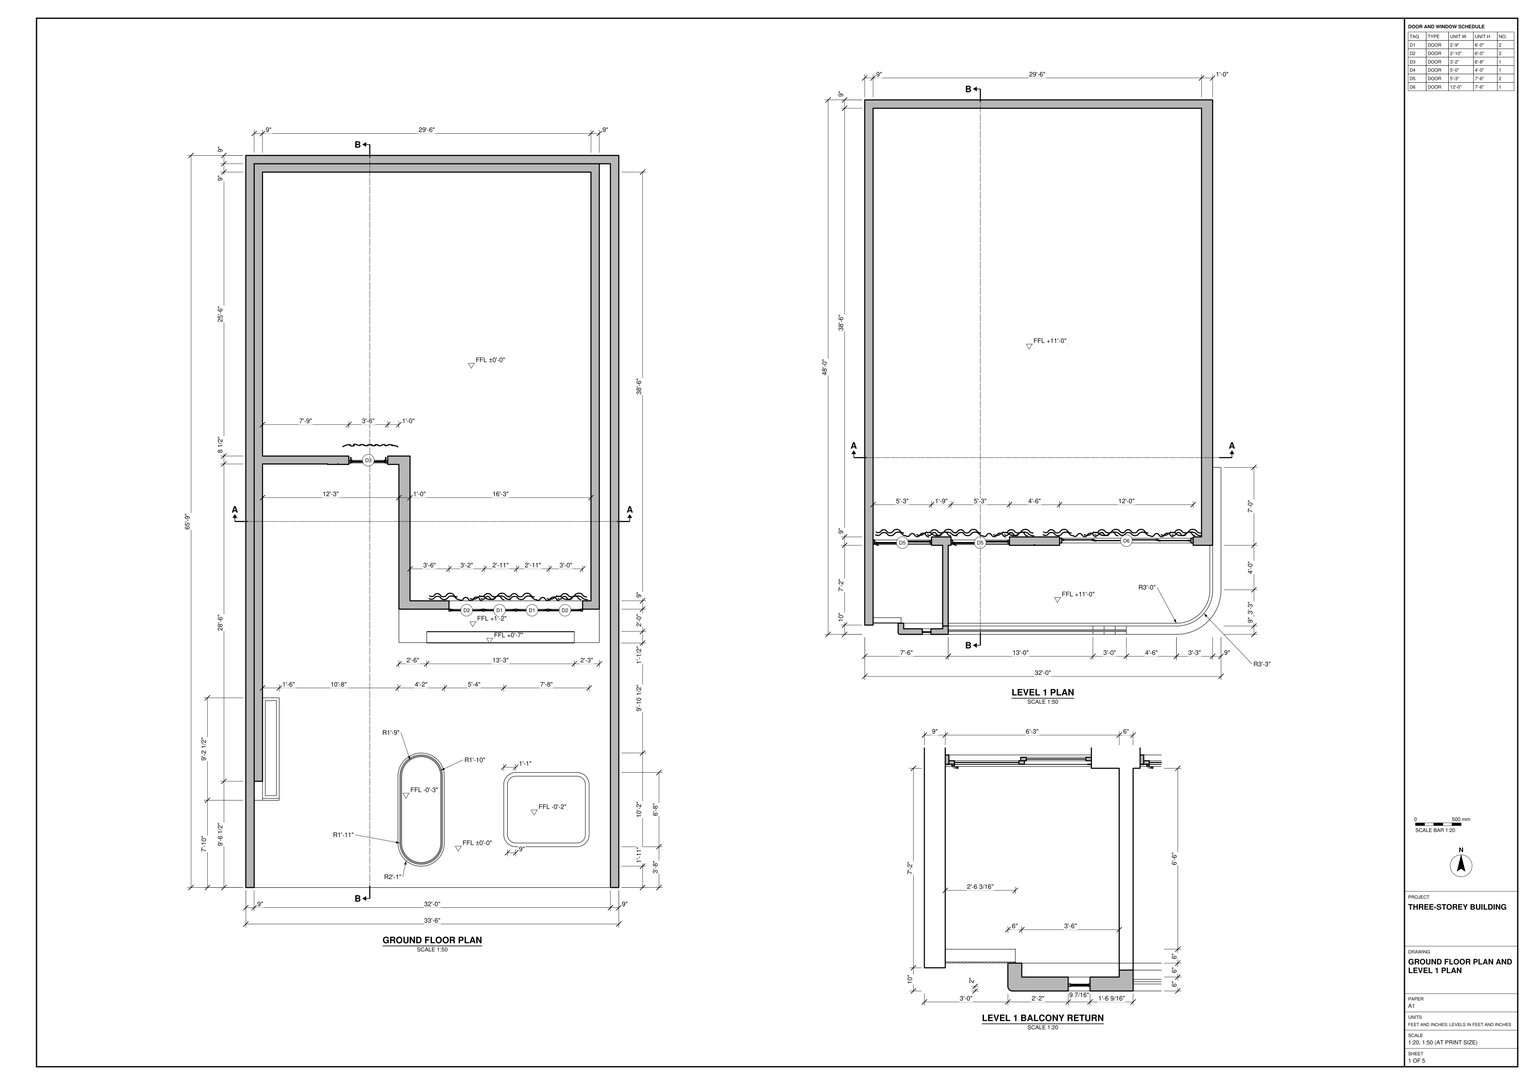
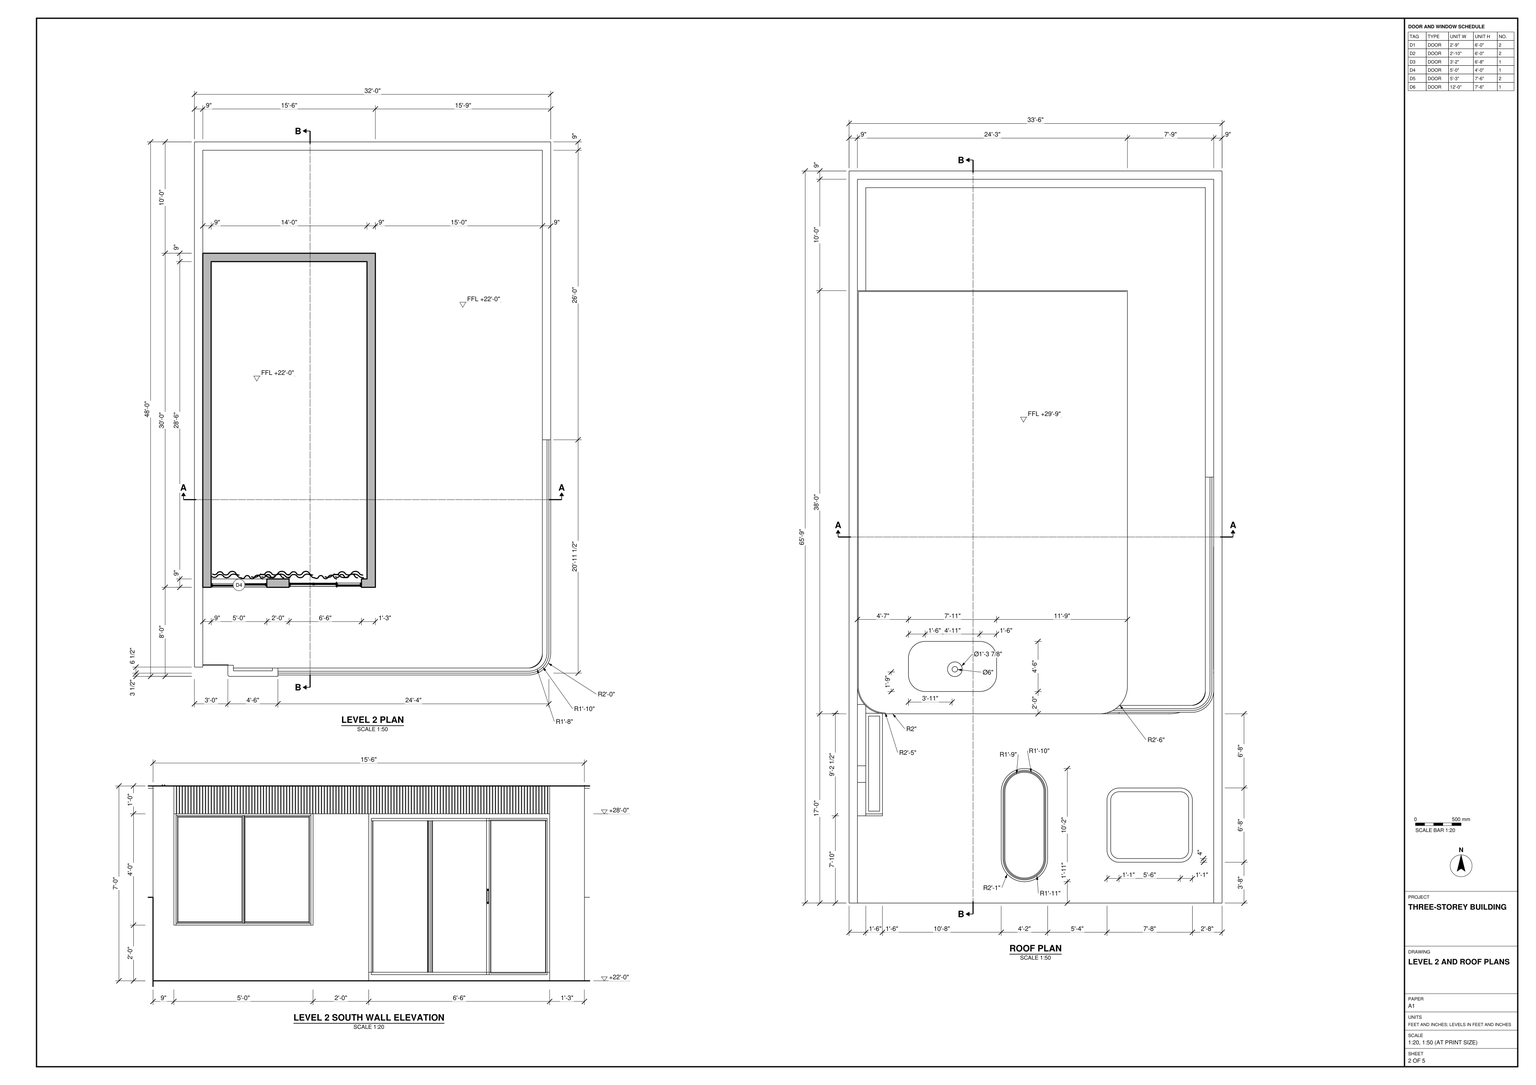
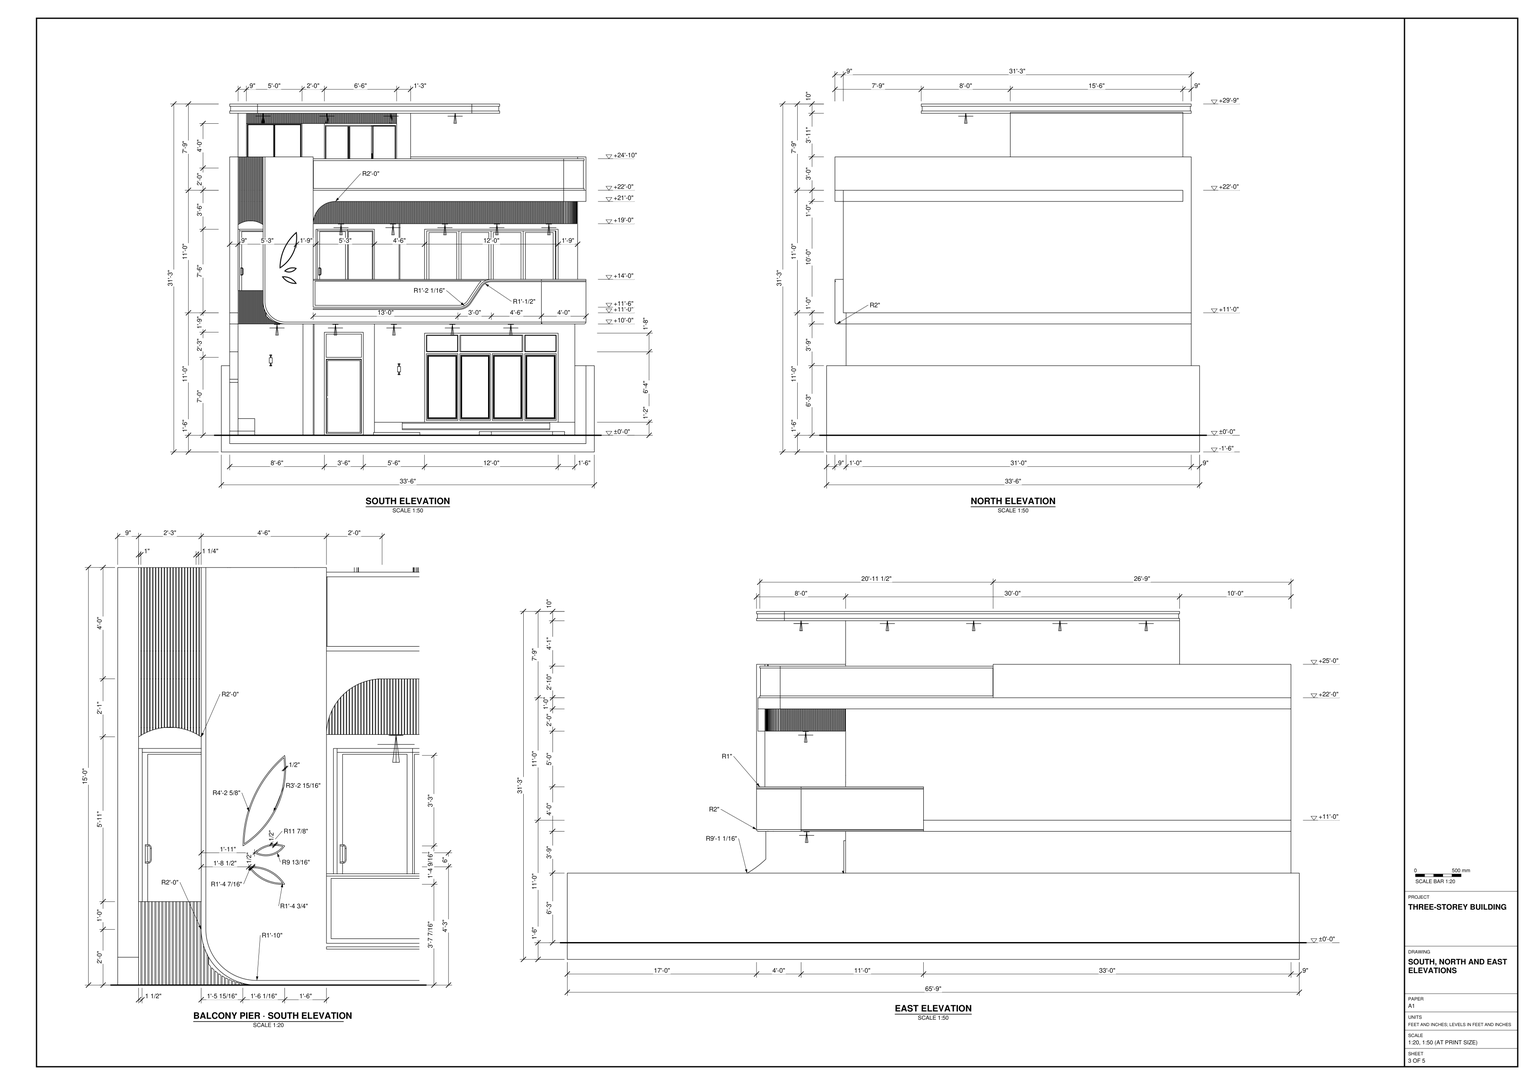
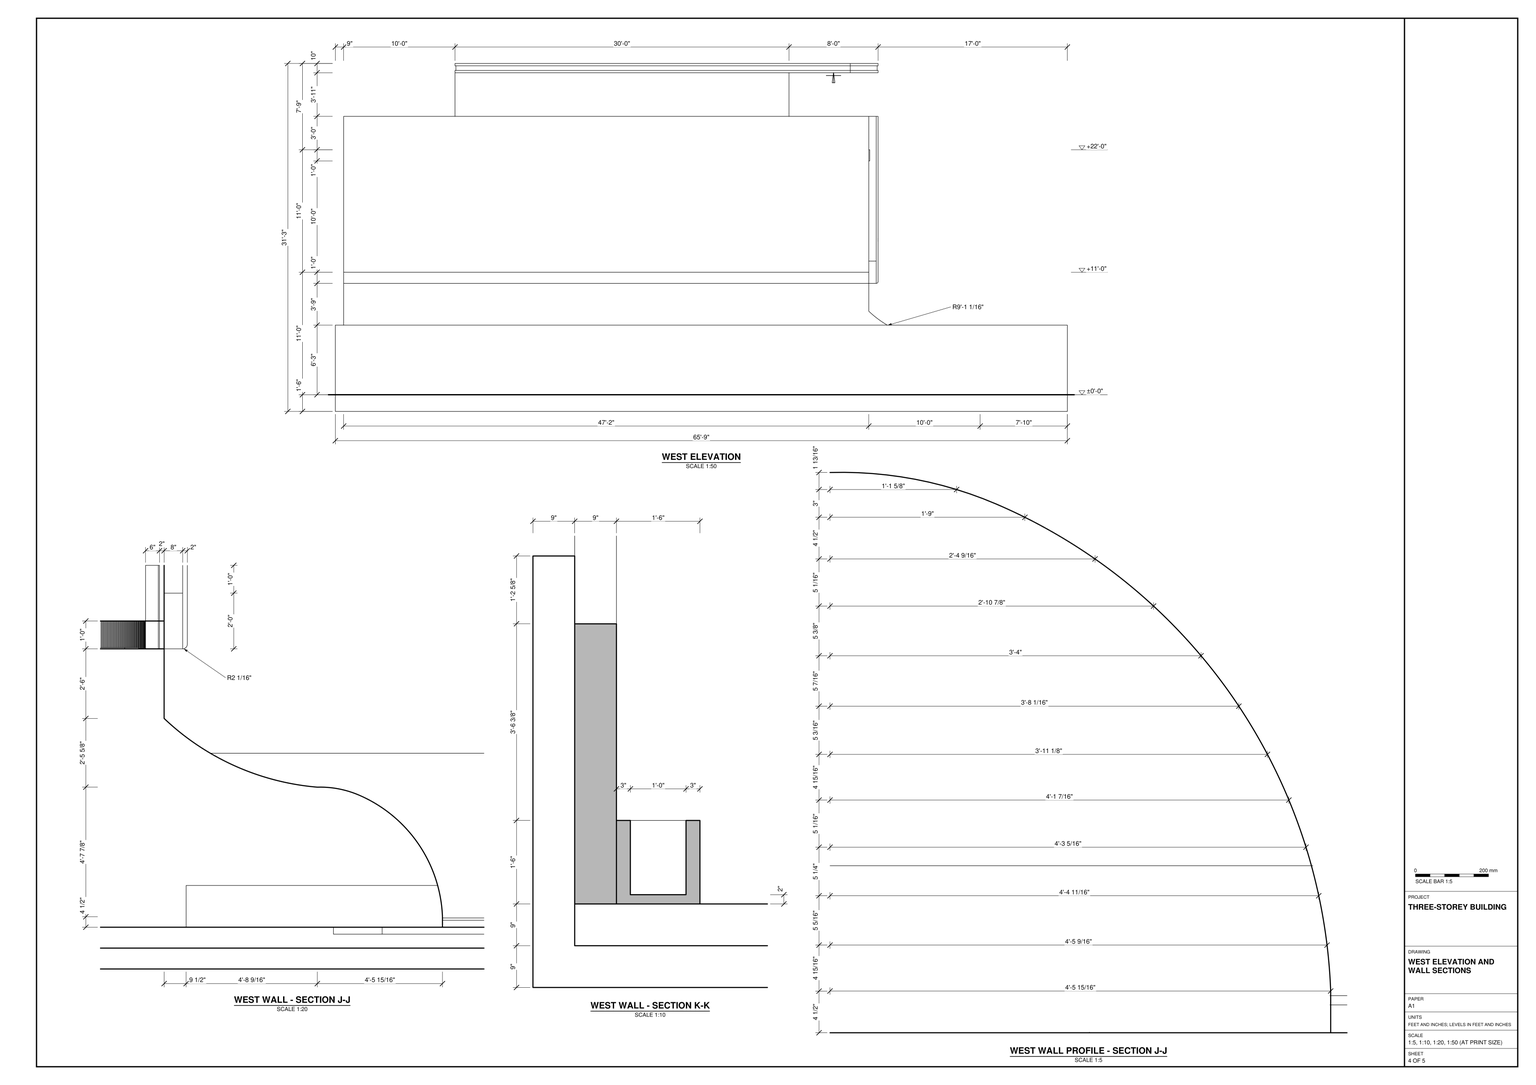
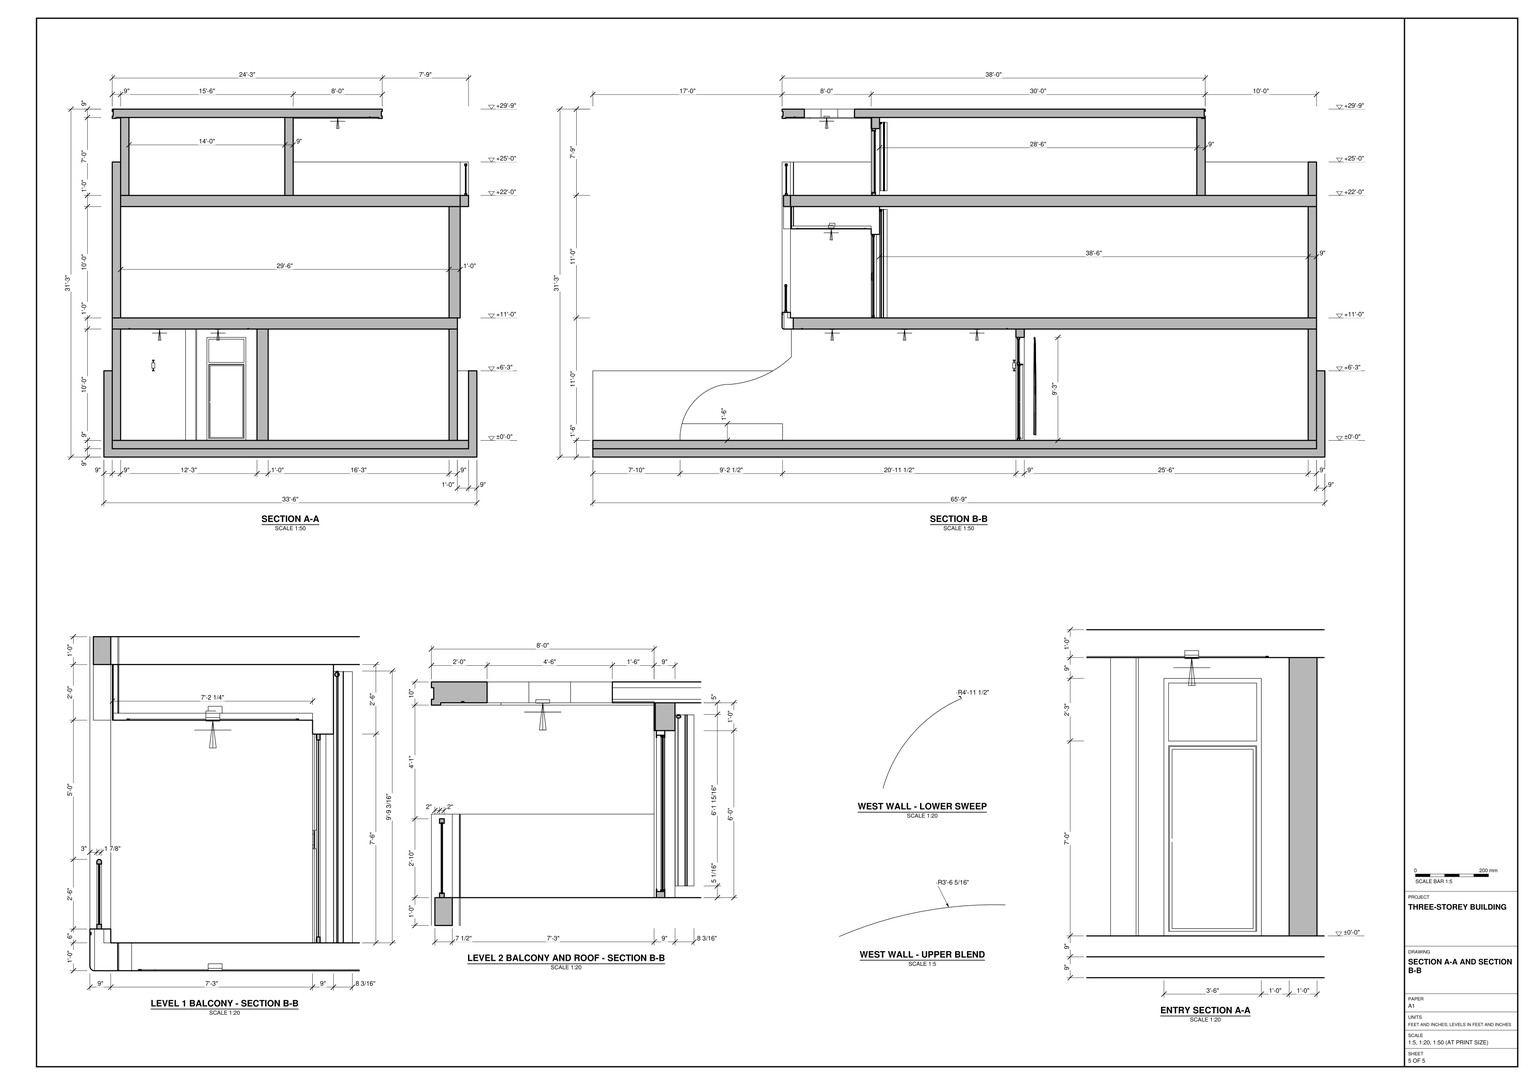
Build the three-storey building in SketchUp from task_files/diagram_01.pdf. Work in feet and inches. The overall dimensions, including the base and forecourt, are 33'-6" wide by 65'-9" deep by 31'-3" high. Set the finished floor levels to ±0'-0", +11'-0" and +22'-0". Include the base below the ground floor so the overall height matches the elevations.

Use the plans to lay out the walls at their drawn thicknesses, including the 9" wall runs and the 1'-0" return beside the recessed entrance. Model the forecourt, its side walls and its rounded inset features. Follow the door schedule and south elevation for the entrance, shallow steps, framed glazing and panels above the ground-floor openings.

At the middle storey, carry the balcony around the rounded front corner and shape its parapet and tall pier from the elevation details. Set the narrower top-storey enclosure back on the terrace and cover it with the projecting flat roof. Use the plans and elevations together to locate slab edges, parapets and openings.

Keep walls, slabs, roof and each furniture or joinery piece shown as separate groups or components, and use components for repeated parts. Decor and loose items may be any suitable library components. Save one SketchUp model as output_files/three_storey_building_curved_balcony_and_roof_terrace.skp.

# SketchUp Ruby script. Lengths in inches.
U = 1.inch
M = Sketchup.active_model
def pt(a) = Geom::Point3d.new(a.map { |v| v * U })
def face(e, loops, mat)
  f = e.add_face(loops[0].map { |a| pt(a) })
  loops[1..].each { |l| e.add_face(l.map { |a| pt(a) }).erase! }
  f.material = f.back_material = mat if mat
  f
end
# faces: each face lists its corners as indices into pts; further lists are holes
def faces(e, pts, list, mat = nil) = list.each { |f| face(e, (f[0].is_a?(Array) ? f : [f]).map { |l| l.map { |i| pts[i] } }, mat) }
# xy, xz, yz: faces in a plane at the given z, y or x. An outline is a flat list of corners, or four numbers for a rectangle; further outlines are holes
def ring(l) = l.size == 4 ? [[l[0], l[1]], [l[2], l[1]], [l[2], l[3]], [l[0], l[3]]] : l.each_slice(2).to_a
def flat(e, list, mat, &to3) = list.each { |f| face(e, (f[0].is_a?(Array) ? f : [f]).map { |l| ring(l).map { |u, v| to3.(u, v) } }, mat) }
def xy(e, z, list, mat = nil) = flat(e, list, mat) { |x, y| [x, y, z] }
def xz(e, y, list, mat = nil) = flat(e, list, mat) { |x, z| [x, y, z] }
def yz(e, x, list, mat = nil) = flat(e, list, mat) { |y, z| [x, y, z] }
def lines(e, pts, list) = list.each { |a, b| e.add_line(pt(pts[a]), pt(pts[b])) }
# prism: a flat outline (further loops are holes) pulled along v
def prism(e, loops, v, mat = nil)
  f = face(e, loops, mat); d = Geom::Vector3d.new(v.map { |x| x * U })
  f.pushpull(f.normal.samedirection?(d) ? d.length : -d.length)
end
def box(e, o, s, mat = nil) = prism(e, [[o, [o[0] + s[0], o[1], o[2]], [o[0] + s[0], o[1] + s[1], o[2]], [o[0], o[1] + s[1], o[2]]]], [0, 0, s[2]], mat)
def at(x, y, z, deg = 0) = Geom::Transformation.translation(pt([x, y, z])) * Geom::Transformation.rotation(ORIGIN, Z_AXIS, deg.degrees)
def axes(o, x, y, z) = Geom::Transformation.new([*x, 0, *y, 0, *z, 0, *pt(o).to_a, 1])
def part(name) = M.definitions.add(name)
# library, detail: a bought-in or finely detailed component or shape, given as its bounding box
def library(name, o, s) = part(name).tap { |d| box(d.entities, o, s) }
def detail(e, o, s) = box(e.add_group.entities, o, s)
def put(e, d, t, mat = nil) = e.add_instance(d, t).tap { |i| i.material = mat if mat }
def group(e, t, mat = nil) = e.add_group.tap { |g| g.transformation = t; g.material = mat if mat }.entities
root = M.entities
M.materials.add("0027 AP L140 CRUSHED ICE").color = [241, 233, 217]
M.materials.add("Black_matte").color = [7, 7, 7]
M.materials.add("Carpet_Frieze_Low").color = [170, 156, 146]
M.materials.add("Carpet_Loop_Low").color = [201, 172, 127]
M.materials.add("Glass_Tinted_Gray").color = [0, 0, 0]
M.materials.add("Glass_headlight").color = [127, 127, 127]
M.materials.add("[0135_DarkGray]").color = [81, 81, 81]
M.materials.add("[Mirror 02]").color = [229, 229, 229]
M.materials.add("[Terrazzo Light Blue]").color = [196, 214, 227]
M.materials.add("[Wood Cherry Original]").color = [103, 58, 28]
c1 = library("CURTAIN",[20.4,9.88,0],[29.77,2.88,102.36])
c2 = library("Sliding glass door",[0,0,0],[5.83,106.3,82.68])
c3 = part("PENTEK_RP Fineline 50S_Sliding_DoorCase_E1")
box(c3.entities,[0,0,0],[1.51,3.66,99.27],"[0135_DarkGray]")
c4 = part("PENTEK_RP Fineline 50S_SlidingDooe_Case_E2")
box(c4.entities,[0,0,0],[96.25,3.66,1.51],"[0135_DarkGray]")
c5 = part("pentek_RP Fineline 50S_SlidingDoor_Case")
put(c5.entities,c3,at(97.76,0,0))
put(c5.entities,c4,at(1.51,0,0))
put(c5.entities,c3,at(0,0,0))
put(c5.entities,c4,at(1.51,0,97.76))
c6 = part("PENTEK_RP Fineline 50S_SlidingDoor_GlazingBead_2")
box(c6.entities,[0,0,0],[0.56,0.59,94.39],"[0135_DarkGray]")
c7 = part("PENTEK_RP Fineline 50S_SlidingDoor_Glass")
box(c7.entities,[0,0,0],[46.58,0.16,94.39],"Glass_Tinted_Gray")
c8 = part("PENTEK_RP Fineline 50S_SlidingDoor_GlazingBead")
box(c8.entities,[0,0,0],[45.47,0.59,0.56],"[0135_DarkGray]")
c9 = part("PENTEK_RP Fineline 50S_SlidingDoor_Leaf_E1")
xy(c9.entities,0,[[0,0,0.93,1.97],[0.93,1.57,1.49,1.97]],"[0135_DarkGray]")
xy(c9.entities,96.25,[[0,0,0.93,0,0.93,1.57,1.49,1.57,1.49,1.97,0,1.97]],"[0135_DarkGray]")
xz(c9.entities,0,[[0,0,0.93,96.25]],"[0135_DarkGray]")
xz(c9.entities,1.57,[[0.93,0,1.49,95.32],[0.93,95.32,1.49,96.25]],"[0135_DarkGray]")
xz(c9.entities,1.97,[[0,0,1.49,96.25]],"[0135_DarkGray]")
yz(c9.entities,0,[[0,0,1.97,96.25]],"[0135_DarkGray]")
yz(c9.entities,0.93,[[0,0,1.57,0.93],[0,0.93,1.57,95.32],[0,95.32,1.57,96.25]],"[0135_DarkGray]")
yz(c9.entities,1.49,[[1.57,0,1.97,95.32],[1.57,95.32,1.97,96.25]],"[0135_DarkGray]")
c10 = part("PENTEK_RP Fineline 50S_SlidingDoor_Leaf_E2")
xy(c10.entities,0,[[0,0,0,1.57,0.56,1.57,0.56,1.97,46.02,1.97,46.02,1.57,46.58,1.57,46.58,0]],"[0135_DarkGray]")
xy(c10.entities,0.93,[[0,0,46.58,1.57]],"[0135_DarkGray]")
xy(c10.entities,1.49,[[0.56,1.57,46.02,1.97]],"[0135_DarkGray]")
xz(c10.entities,0,[[0,0,46.58,0.93]],"[0135_DarkGray]")
xz(c10.entities,1.57,[[0,0,0.56,0.93],[46.02,0,46.58,0.93],[0.56,0.93,46.02,1.49]],"[0135_DarkGray]")
xz(c10.entities,1.97,[[0.56,0,46.02,1.49]],"[0135_DarkGray]")
yz(c10.entities,0,[[0,0,1.57,0.93]],"[0135_DarkGray]")
yz(c10.entities,0.56,[[1.57,0,1.97,0.93],[1.57,0.93,1.97,1.49]],"[0135_DarkGray]")
yz(c10.entities,46.02,[[1.57,0,1.97,0.93],[1.57,0.93,1.97,1.49]],"[0135_DarkGray]")
yz(c10.entities,46.58,[[0,0,1.57,0.93]],"[0135_DarkGray]")
c11 = part("PENTEK_RP Fineline S_SlidingDoor_Leaf1")
put(c11.entities,c6,at(0.93,0,0.93))
put(c11.entities,c6,at(46.96,0,0.93))
put(c11.entities,c7,at(1.49,1.42,0.93))
put(c11.entities,c8,at(1.49,0,0.93))
put(c11.entities,c7,at(1.49,0.59,0.93),"[Terrazzo Light Blue]")
put(c11.entities,c9,at(0,0,0))
put(c11.entities,c9,axes([48.44,0,0],[-1,0,0],[0,1,0],[0,0,1]))
put(c11.entities,c10,axes([0.93,0,96.25],[1,0,0],[0,1,0],[0,0,-1]))
put(c11.entities,c10,at(0.93,0,0))
put(c11.entities,c8,at(1.49,0,94.77))
c12 = part("PENTEK_RP Fineline 50S_SlidingDoor_Leaf2")
put(c12.entities,c7,at(1.49,1.42,0.93))
put(c12.entities,c8,at(1.49,0,94.77))
put(c12.entities,c6,at(46.96,0,0.93))
put(c12.entities,c7,at(1.49,0.59,0.93),"[Mirror 02]")
put(c12.entities,c6,at(0.93,0,0.93))
put(c12.entities,c9,at(0,0,0))
put(c12.entities,c9,axes([48.44,0,0],[-1,0,0],[0,1,0],[0,0,1]))
put(c12.entities,c8,at(1.49,0,0.93))
put(c12.entities,c10,axes([0.93,0,96.25],[1,0,0],[0,1,0],[0,0,-1]))
put(c12.entities,c10,at(0.93,0,0))
c13 = part("PENTEK - Slimmest Steel Sliding Door / Window\#1")
put(c13.entities,c5,at(0,-1.88,-0.09))
put(c13.entities,c11,at(1.51,-2.27,1.42))
put(c13.entities,c12,at(49.32,-0.3,1.42))
c14 = library("Wheel1",[-0.22,0.28,-1.22],[12.14,34.32,34.67])
c15 = library("Group\#47",[0,0,0],[81,26.91,31.48])
c16 = library("Group\#46",[0,-11.74,0],[75.48,151.34,31.8125])
c17 = library("Group\#45",[0,0,0],[59.24,11.61,17.61])
c18 = library("Group\#48",[0,0,0],[83.57,167.11,42.22])
c19 = library("Group\#49",[0,0,0],[97.91,11.39,8.3])
c20 = library("Group\#50",[0,0,0],[82.49,206.98,67.77])
c21 = library("Group\#51",[0,0,0],[82.02,206.91,71.71])
c22 = part("l405 Vogue 2013")
put(c22.entities,c14,axes([23.09,177.11,0.71],[-1.08,0,0],[0,-1,0],[0,0,1]))
put(c22.entities,c14,axes([83.66,53.48,1.89],[1.08,0,0],[0,-1,0],[0,0,1]))
put(c22.entities,c14,axes([23.09,53.48,1.89],[-1.08,0,0],[0,-1,0],[0,0,1]))
put(c22.entities,c14,axes([83.66,177.11,0.71],[1.08,0,0],[0,-1,0],[0,0,1]))
put(c22.entities,c15,axes([97.16,27.0625,11.6],[-1.08,0,0],[0,-1,0],[0,0,1]))
put(c22.entities,c16,axes([94.18,192.03,48.94],[-1.08,0,0],[0,-1,0],[0,0,1]),"Glass_headlight")
put(c22.entities,c17,axes([85.41,206.68,30.35],[-1.08,0,0],[0,-1,0],[0,0,1]))
put(c22.entities,c18,axes([98.55,177.66,12.76],[-1.08,0,0],[0,-1,0],[0,0,1]))
put(c22.entities,c19,axes([106.29,85.5,53.72],[-1.08,0,0],[0,-1,0],[0,0,1]))
put(c22.entities,c20,axes([97.96,207.84,12.8],[-1.08,0,0],[0,-1,0],[0,0,1]))
put(c22.entities,c21,axes([97.7,207.32,9.05],[-1.08,0,0],[0,-1,0],[0,0,1]))
c23 = part("2013 Land Rover Range Rover l405")
put(c23.entities,c22,axes([0,0,0],[1,0,0],[0,1.03,0],[0,0,1]),"Black_matte")
c24 = part("2014+Range+Rover+l405+UK-version+ISA")
put(c24.entities,c23,at(0,0,0),"Black_matte")
c25 = library("Group\#2",[0,-206,0],[372,686,120])
c26 = library("Group\#11",[0,-90,0],[384,570,168])
c27 = library("Group\#22",[-9,-309,-9],[384,780,13])
c28 = library("Group\#32",[0,-3.5,0],[366,567,12])
c29 = library("Group\#21",[0,-96,-12.07],[384,576,192.07])
c30 = part("Curtain panel")
# 43 loose lines left out
p = [[17.625,0.0625,78.74],[17.625,0.0625,0],[18.27,0,0],[18.27,0,78.74],[18.92,0.0625,0],[18.92,0.0625,78.74],
  [17,0.25,78.74],[17,0.25,0],[19.55,0.25,0],[19.55,0.25,78.74],[16.43,0.56,78.74],[16.43,0.56,0],
  [20.12,0.56,0],[20.12,0.56,78.74],[6.31,0.6,78.74],[6.31,0.6,0],[6.8125,0.45,0],[6.8125,0.45,78.74],
  [7.33,0.4,0],[7.33,0.4,78.74],[7.86,0.45,0],[7.86,0.45,78.74],[8.36,0.6,0],[8.36,0.6,78.74],
  [5.85,0.85,78.74],[5.85,0.85,0],[8.82,0.85,0],[8.82,0.85,78.74],[15.92,0.97,78.74],[15.92,0.97,0],
  [20.625,0.97,0],[20.625,0.97,78.74],[5.44,1.18,78.74],[5.44,1.18,0],[9.23,1.18,0],[9.23,1.18,78.74],
  [15.51,1.48,78.74],[15.51,1.48,0],[21.04,1.48,0],[21.04,1.48,78.74],[5.11,1.59,78.74],[5.11,1.59,0],
  [9.5625,1.59,0],[9.5625,1.59,78.74],[14.93,2.55,78.74],[14.93,2.55,0],[15.2,2.04,0],[15.2,2.04,78.74],
  [21.34,2.04,0],[21.64,2.59,0],[21.64,2.59,78.74],[21.34,2.04,78.74],[4.63,2.47,78.74],[4.63,2.47,0],
  [4.86,2.04,0],[4.86,2.04,78.74],[9.81,2.04,0],[10.08,2.55,0],[10.08,2.55,78.74],[9.81,2.04,78.74],
  [4.32,2.85,78.74],[4.32,2.85,0],[10.44,2.99,0],[10.44,2.99,78.74],[14.57,2.99,78.74],[14.57,2.99,0],
  [22.03,3.0625,0],[22.03,3.0625,78.74],[0.85,2.85,78.74],[0.85,2.85,0],[1.22,3.15,0],[1.22,3.15,78.74],
  [3.95,3.15,78.74],[3.95,3.15,0],[10.89,3.35,0],[10.89,3.35,78.74],[14.125,3.35,78.74],[14.125,3.35,0],
  [22.5,3.45,0],[22.5,3.45,78.74],[1.65,3.375,0],[1.65,3.375,78.74],[3.53,3.375,78.74],[3.53,3.375,0],
  [2.11,3.52,0],[2.11,3.52,78.74],[3.07,3.52,78.74],[3.07,3.52,0],[11.39,3.625,0],[11.39,3.625,78.74],
  [13.62,3.625,78.74],[13.62,3.625,0],[2.59,3.5625,0],[2.59,3.5625,78.74],[23.04,3.74,0],[23.04,3.74,78.74],
  [11.9375,3.79,0],[11.9375,3.79,78.74],[13.07,3.79,78.74],[13.07,3.79,0],[23.63,3.92,0],[23.63,3.92,78.74],
  [12.51,3.85,0],[12.51,3.85,78.74],[24.25,3.98,0],[24.25,3.98,78.74]]
faces(c30.entities,p,[[0,1,2,3],[3,2,4,5],[6,7,1,0],[5,4,8,9],[10,11,7,6],[9,8,12,13],[14,15,16,17],[17,16,18,19],
  [19,18,20,21],[21,20,22,23],[24,25,15,14],[23,22,26,27],[28,29,11,10],[13,12,30,31],[32,33,25,24],[27,26,34,35],
  [36,37,29,28],[31,30,38,39],[40,41,33,32],[35,34,42,43],[44,45,46,37,36,47],[39,38,48,49,50,51],[52,53,54,41,40,55],[43,42,56,57,58,59],
  [60,61,53,52],[58,57,62,63],[64,65,45,44],[50,49,66,67],[68,69,70,71],[72,73,61,60],[63,62,74,75],[76,77,65,64],
  [67,66,78,79],[71,70,80,81],[82,83,73,72],[81,80,84,85],[86,87,83,82],[75,74,88,89],[90,91,77,76],[85,84,92,93],
  [93,92,87,86],[79,78,94,95],[89,88,96,97],[98,99,91,90],[95,94,100,101],[97,96,102,103],[103,102,99,98],[101,100,104,105]])
c31 = part("Rod section")
yz(c31.entities,0,[[1.55,0.61,1.31,0.64,1.08,0.73,0.88,0.88,0.73,1.08,0.64,1.31,0.61,1.55,0.64,1.79,0.73,2.02,0.88,2.22,1.08,2.37,1.31,2.46,1.55,2.49,1.79,2.46,2.02,2.37,2.22,2.22,2.37,2.02,2.46,1.79,2.49,1.55,2.46,1.31,2.37,1.08,2.22,0.88,2.02,0.73,1.79,0.64]])
yz(c31.entities,2.36,[[[1.55,0,1.15,0.05,0.78,0.21,0.45,0.45,0.21,0.78,0.05,1.15,0,1.55,0.05,1.95,0.21,2.33,0.45,2.65,0.78,2.89,1.15,3.05,1.55,3.1,1.95,3.05,2.33,2.89,2.65,2.65,2.89,2.33,3.05,1.95,3.1,1.55,3.05,1.15,2.89,0.78,2.65,0.45,2.33,0.21,1.95,0.05],[1.55,0.61,1.79,0.64,2.02,0.73,2.22,0.88,2.37,1.08,2.46,1.31,2.49,1.55,2.46,1.79,2.37,2.02,2.22,2.22,2.02,2.37,1.79,2.46,1.55,2.49,1.31,2.46,1.08,2.37,0.88,2.22,0.73,2.02,0.64,1.79,0.61,1.55,0.64,1.31,0.73,1.08,0.88,0.88,1.08,0.73,1.31,0.64]]])
yz(c31.entities,3.15,[[[1.55,0,1.95,0.05,2.33,0.21,2.65,0.45,2.89,0.78,3.05,1.15,3.1,1.55,3.05,1.95,2.89,2.33,2.65,2.65,2.33,2.89,1.95,3.05,1.55,3.1,1.15,3.05,0.78,2.89,0.45,2.65,0.21,2.33,0.05,1.95,0,1.55,0.05,1.15,0.21,0.78,0.45,0.45,0.78,0.21,1.15,0.05],[1.55,0.61,1.31,0.64,1.08,0.73,0.88,0.88,0.73,1.08,0.64,1.31,0.61,1.55,0.64,1.79,0.73,2.02,0.88,2.22,1.08,2.37,1.31,2.46,1.55,2.49,1.79,2.46,2.02,2.37,2.22,2.22,2.37,2.02,2.46,1.79,2.49,1.55,2.46,1.31,2.37,1.08,2.22,0.88,2.02,0.73,1.79,0.64]]])
yz(c31.entities,61.24,[[1.55,0.61,1.79,0.64,2.02,0.73,2.22,0.88,2.37,1.08,2.46,1.31,2.49,1.55,2.46,1.79,2.37,2.02,2.22,2.22,2.02,2.37,1.79,2.46,1.55,2.49,1.31,2.46,1.08,2.37,0.88,2.22,0.73,2.02,0.64,1.79,0.61,1.55,0.64,1.31,0.73,1.08,0.88,0.88,1.08,0.73,1.31,0.64]])
p = [[2.36,1.15,0.05],[2.36,1.55,0],[3.15,1.55,0],[3.15,1.15,0.05],[2.36,1.95,0.05],[3.15,1.95,0.05],
  [2.36,0.78,0.21],[3.15,0.78,0.21],[2.36,2.33,0.21],[3.15,2.33,0.21],[2.36,0.45,0.45],[3.15,0.45,0.45],
  [2.36,2.65,0.45],[3.15,2.65,0.45],[2.36,0.21,0.78],[3.15,0.21,0.78],[2.36,2.89,0.78],[3.15,2.89,0.78],
  [2.36,1.31,0.64],[2.36,1.08,0.73],[0,1.08,0.73],[0,1.31,0.64],[3.15,1.31,0.64],[3.15,1.08,0.73],
  [61.24,1.31,0.64],[61.24,1.08,0.73],[2.36,1.55,0.61],[0,1.55,0.61],[3.15,1.55,0.61],[61.24,1.55,0.61],
  [2.36,1.79,0.64],[0,1.79,0.64],[3.15,1.79,0.64],[61.24,1.79,0.64],[2.36,2.02,0.73],[0,2.02,0.73],
  [3.15,2.02,0.73],[61.24,2.02,0.73],[2.36,0.88,0.88],[0,0.88,0.88],[3.15,0.88,0.88],[61.24,0.88,0.88],
  [2.36,2.22,0.88],[0,2.22,0.88],[3.15,2.22,0.88],[61.24,2.22,0.88],[2.36,0.05,1.15],[3.15,0.05,1.15],
  [2.36,3.05,1.15],[3.15,3.05,1.15],[2.36,0.73,1.08],[0,0.73,1.08],[3.15,0.73,1.08],[61.24,0.73,1.08],
  [2.36,2.37,1.08],[0,2.37,1.08],[3.15,2.37,1.08],[61.24,2.37,1.08],[2.36,0,1.55],[3.15,0,1.55],
  [2.36,0.64,1.31],[0,0.64,1.31],[3.15,0.64,1.31],[61.24,0.64,1.31],[2.36,2.46,1.31],[0,2.46,1.31],
  [3.15,2.46,1.31],[61.24,2.46,1.31],[2.36,3.1,1.55],[3.15,3.1,1.55],[2.36,0.61,1.55],[0,0.61,1.55],
  [3.15,0.61,1.55],[61.24,0.61,1.55],[2.36,2.49,1.55],[0,2.49,1.55],[3.15,2.49,1.55],[61.24,2.49,1.55],
  [2.36,0.05,1.95],[3.15,0.05,1.95],[2.36,0.64,1.79],[0,0.64,1.79],[3.15,0.64,1.79],[61.24,0.64,1.79],
  [2.36,2.46,1.79],[0,2.46,1.79],[3.15,2.46,1.79],[61.24,2.46,1.79],[2.36,3.05,1.95],[3.15,3.05,1.95],
  [2.36,0.73,2.02],[0,0.73,2.02],[3.15,0.73,2.02],[61.24,0.73,2.02],[2.36,2.37,2.02],[0,2.37,2.02],
  [3.15,2.37,2.02],[61.24,2.37,2.02],[2.36,0.21,2.33],[3.15,0.21,2.33],[2.36,0.88,2.22],[0,0.88,2.22],
  [3.15,0.88,2.22],[61.24,0.88,2.22],[2.36,2.22,2.22],[0,2.22,2.22],[3.15,2.22,2.22],[61.24,2.22,2.22],
  [2.36,2.89,2.33],[3.15,2.89,2.33],[2.36,1.08,2.37],[0,1.08,2.37],[3.15,1.08,2.37],[61.24,1.08,2.37],
  [2.36,2.02,2.37],[0,2.02,2.37],[3.15,2.02,2.37],[61.24,2.02,2.37],[2.36,0.45,2.65],[3.15,0.45,2.65],
  [2.36,2.65,2.65],[3.15,2.65,2.65],[2.36,1.31,2.46],[0,1.31,2.46],[3.15,1.31,2.46],[61.24,1.31,2.46],
  [2.36,1.79,2.46],[0,1.79,2.46],[3.15,1.79,2.46],[61.24,1.79,2.46],[2.36,1.55,2.49],[0,1.55,2.49],
  [3.15,1.55,2.49],[61.24,1.55,2.49],[2.36,0.78,2.89],[3.15,0.78,2.89],[2.36,2.33,2.89],[3.15,2.33,2.89],
  [2.36,1.15,3.05],[3.15,1.15,3.05],[2.36,1.95,3.05],[3.15,1.95,3.05],[2.36,1.55,3.1],[3.15,1.55,3.1]]
faces(c31.entities,p,[[0,1,2,3],[1,4,5,2],[6,0,3,7],[4,8,9,5],[10,6,7,11],[8,12,13,9],[14,10,11,15],[12,16,17,13],
  [18,19,20,21],[19,18,22,23],[24,25,23,22],[26,18,21,27],[18,26,28,22],[29,24,22,28],[30,26,27,31],[26,30,32,28],
  [33,29,28,32],[34,30,31,35],[30,34,36,32],[37,33,32,36],[19,38,39,20],[38,19,23,40],[25,41,40,23],[42,34,35,43],
  [34,42,44,36],[45,37,36,44],[46,14,15,47],[16,48,49,17],[38,50,51,39],[50,38,40,52],[41,53,52,40],[54,42,43,55],
  [42,54,56,44],[57,45,44,56],[58,46,47,59],[50,60,61,51],[60,50,52,62],[53,63,62,52],[64,54,55,65],[54,64,66,56],
  [67,57,56,66],[48,68,69,49],[60,70,71,61],[70,60,62,72],[63,73,72,62],[74,64,65,75],[64,74,76,66],[77,67,66,76],
  [78,58,59,79],[70,80,81,71],[80,70,72,82],[73,83,82,72],[84,74,75,85],[74,84,86,76],[87,77,76,86],[68,88,89,69],
  [80,90,91,81],[90,80,82,92],[83,93,92,82],[94,84,85,95],[84,94,96,86],[97,87,86,96],[98,78,79,99],[90,100,101,91],
  [100,90,92,102],[93,103,102,92],[104,94,95,105],[94,104,106,96],[107,97,96,106],[88,108,109,89],[100,110,111,101],[110,100,102,112],
  [103,113,112,102],[114,104,105,115],[104,114,116,106],[117,107,106,116],[118,98,99,119],[108,120,121,109],[110,122,123,111],[122,110,112,124],
  [113,125,124,112],[126,114,115,127],[114,126,128,116],[129,117,116,128],[122,130,131,123],[130,122,124,132],[125,133,132,124],[130,126,127,131],
  [126,130,132,128],[133,129,128,132],[134,118,119,135],[120,136,137,121],[138,134,135,139],[136,140,141,137],[142,138,139,143],[140,142,143,141]])
c32 = part("Curtain rod")
put(c32.entities,c31,axes([3.125,-0.76,-71.54],[0,0,1.25313],[0,1.25313,0],[-1.25313,0,0]))
put(c32.entities,c31,axes([3.125,3.125,81],[0,0,-1.25313],[0,-1.25313,0],[-1.25313,0,0]))
c33 = part("Group\#61")
put(c33.entities,c30,axes([-0.76,0,0],[0.8979,0,0],[0,1,0],[0,0,1]),"Carpet_Frieze_Low")
put(c33.entities,c30,axes([37.23,0,0],[0.9782,0,0],[0,1,0],[0,0,1]),"Carpet_Frieze_Low")
c34 = part("curtain2")
p = [[59.99,12.8,78.74],[59.99,12.8,-38.1875],[60.15,12.52,-38.1875],[60.15,12.52,78.74],[66.72,13.7,-38.1875],[66.72,13.7,78.74],
  [73.91,13.97,78.74],[73.91,13.97,-38.1875],[49.31,14.13,-38.1875],[49.31,14.13,78.74],[2.67,12.52,-38.1875],[2.67,12.52,78.74],
  [-8.17,14.13,-38.1875],[-8.17,14.13,78.74],[2.51,12.8,78.74],[2.51,12.8,-38.1875],[16.42,13.97,78.74],[16.42,13.97,-38.1875],
  [9.24,13.7,-38.1875],[9.24,13.7,78.74]]
lines(c34.entities,p,[[0,1],[2,3],[4,5],[6,7],[8,9],[10,11],[12,13],[14,15],[16,17],[18,19]])
put(c34.entities,c30,axes([64.94,10.15,-38.1875],[0.73,0,0],[0,1,0],[0,0,1.485]),"Carpet_Loop_Low")
put(c34.entities,c30,axes([48.6875,11.28,-38.1875],[0.73,0,0],[0,1,0],[0,0,1.485]),"Carpet_Loop_Low")
put(c34.entities,c30,axes([25.83,10.15,-38.1875],[0.96815,0,0],[0,1,0],[0,0,1.485]),"Carpet_Loop_Low")
put(c34.entities,c30,axes([56.28,10.09,-38.1875],[1.28298,0,0],[0,1,0],[0,0,1.485]),"Carpet_Loop_Low")
put(c34.entities,c32,axes([25.47,12.88,78.42],[0,0,-0.798],[0,0.798,0],[0.798,0,0]))
put(c34.entities,c30,axes([7.46,10.15,-38.1875],[0.73,0,0],[0,1,0],[0,0,1.485]),"Carpet_Loop_Low")
put(c34.entities,c30,axes([-1.2,10.09,-38.1875],[1.28298,0,0],[0,1,0],[0,0,1.485]),"Carpet_Loop_Low")
put(c34.entities,c30,axes([-8.79,11.28,-38.1875],[0.73,0,0],[0,1,0],[0,0,1.485]),"Carpet_Loop_Low")
put(c34.entities,c30,axes([-31.65,10.15,-38.1875],[0.96815,0,0],[0,1,0],[0,0,1.485]),"Carpet_Loop_Low")
put(c34.entities,c33,axes([27.05,7.18,-38.1875],[0.98,0,0],[0,1,0],[0,0,1.485]))
put(c34.entities,c33,axes([-30.43,7.18,-38.1875],[0.98,0,0],[0,1,0],[0,0,1.485]))
c35 = part("Curtains")
put(c35.entities,c34,axes([31.62,15.375,38.1875],[1,0,0],[0,-1,0],[0,0,1]))
c36 = library("Group419\#1",[-81,-6,0],[162,12,0.5])
c37 = library("Group\#40",[-9,-96,-10.82],[291,456,20.82])
put(root,c1,axes([63.62,465,5.93],[2,0,0],[0,1,0],[0,0,1.03]))
g1 = group(root,at(9,300,0))
put(g1,c2,axes([180,0,264],[0,1,0],[-0.73378,0,0],[0,0,0.87087]))
put(g1,c13,axes([18,2.77,288.04],[0.6044,0,0],[0,0.7182,0],[0,0,0.48352]))
put(g1,c24,axes([33.78,-142,-0.07],[0.8184,0,0],[0,0.91,0],[0,0,0.86765]))
put(g1,c25,at(0,0,0),"0027 AP L140 CRUSHED ICE")
put(g1,c26,at(0,0,132))
put(g1,c27,at(9,9,0))
put(g1,c28,at(9,-83.5,252))
put(g1,c29,at(0,0,120),"0027 AP L140 CRUSHED ICE")
g2 = group(g1,at(9,0,264),"0027 AP L140 CRUSHED ICE")
xy(g2,0,[[0,0,0,360,186,360,186,0,171,0,171,9,177,9,177,351,9,351,9,9,93,9,93,0]])
xy(g2,24,[[9,0,69,9]])
xy(g2,72,[[69,0,93,0.5],[9,0.5,69,9],[93,0.5,171,9]])
xy(g2,84,[[[0,0,9,0,9,0.5,171,0.5,171,0,186,0,186,360,0,360],[9,9,177,351]]])
xz(g2,0,[[0,0,93,0,93,72,69,72,69,24,9,24,9,84,0,84],[171,0,186,84]])
xz(g2,0.5,[[9,72,171,84]])
xz(g2,9,[[9,0,9,24,69,24,69,72,9,72,9,84,177,84,177,0,171,0,171,72,93,72,93,0]])
xz(g2,351,[[9,0,177,84]])
xz(g2,360,[[0,0,186,84]])
yz(g2,0,[[0,0,360,84]])
yz(g2,9,[[9,0,351,84],[0,24,9,72],[0,72,0.5,84]])
yz(g2,69,[[0,24,9,72]])
yz(g2,93,[[0,0,9,72]])
yz(g2,171,[[0,0,9,72],[0,72,0.5,84]])
yz(g2,177,[[9,0,351,84]])
yz(g2,186,[[0,0,360,84]])
put(g2,c35,axes([9,9,5.06],[1.38014,0,0],[0,1,0],[0,0,0.63062]))
g3 = group(g2,at(9,0.5,72),"[Wood Cherry Original]")
put(g3,c36,axes([81,0,6],[1,0,0],[0,0,1],[0,-1,0]))
put(g1,c37,at(9,0,347))
g4 = group(g1,at(0,-300,-9))
xy(g4,-9,[[-9,0,393,789]])
xy(g4,0,[[0,0,384,780]])
xy(g4,84,[[-9,0,0,0,0,780,384,780,384,0,393,0,393,789,-9,789]])
xz(g4,0,[[-9,-9,393,-9,393,84,384,84,384,0,0,0,0,84,-9,84]])
xz(g4,780,[[0,0,384,84]])
xz(g4,789,[[-9,-9,393,84]])
yz(g4,-9,[[0,-9,789,84]])
yz(g4,0,[[0,0,780,84]])
yz(g4,384,[[0,0,780,84]])
yz(g4,393,[[0,-9,789,84]])
